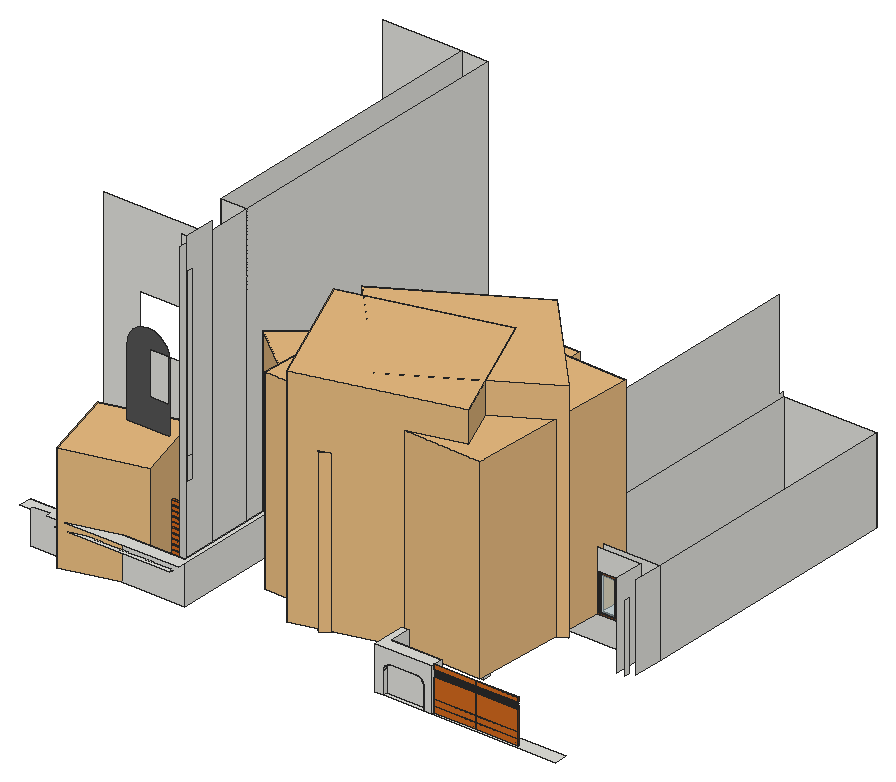
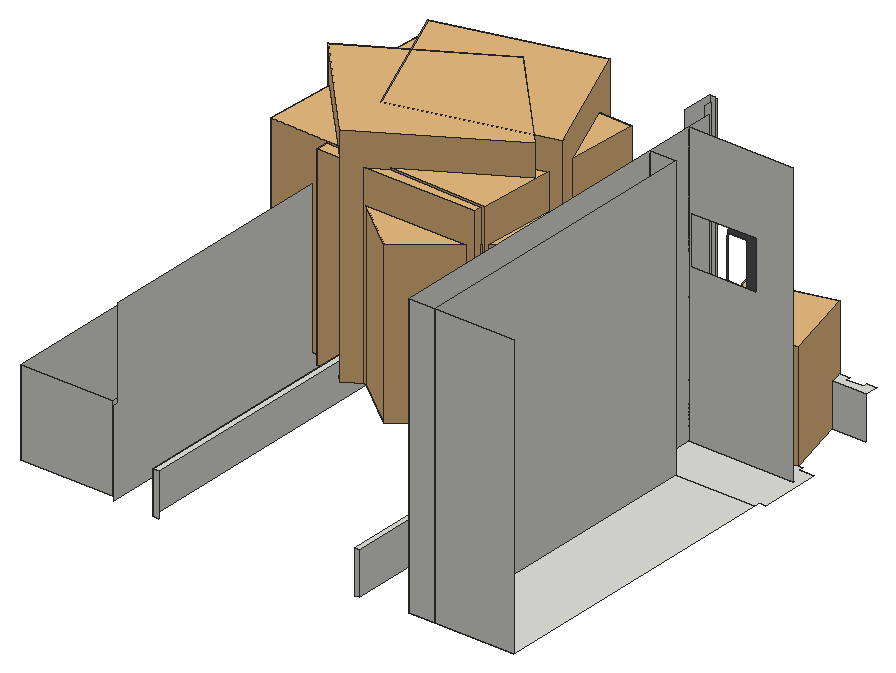
# SketchUp Ruby script. Lengths in inches.
U = 1.inch
M = Sketchup.active_model
def pt(a) = Geom::Point3d.new(a.map { |v| v * U })
def face(e, loops, mat)
  f = e.add_face(loops[0].map { |a| pt(a) })
  loops[1..].each { |l| e.add_face(l.map { |a| pt(a) }).erase! }
  f.material = f.back_material = mat if mat
  f
end
# faces: each face lists its corners as indices into pts; further lists are holes
def faces(e, pts, list, mat = nil) = list.each { |f| face(e, (f[0].is_a?(Array) ? f : [f]).map { |l| l.map { |i| pts[i] } }, mat) }
# xy, xz, yz: faces in a plane at the given z, y or x. An outline is a flat list of corners, or four numbers for a rectangle; further outlines are holes
def ring(l) = l.size == 4 ? [[l[0], l[1]], [l[2], l[1]], [l[2], l[3]], [l[0], l[3]]] : l.each_slice(2).to_a
def flat(e, list, mat, &to3) = list.each { |f| face(e, (f[0].is_a?(Array) ? f : [f]).map { |l| ring(l).map { |u, v| to3.(u, v) } }, mat) }
def xy(e, z, list, mat = nil) = flat(e, list, mat) { |x, y| [x, y, z] }
def xz(e, y, list, mat = nil) = flat(e, list, mat) { |x, z| [x, y, z] }
def yz(e, x, list, mat = nil) = flat(e, list, mat) { |y, z| [x, y, z] }
def lines(e, pts, list) = list.each { |a, b| e.add_line(pt(pts[a]), pt(pts[b])) }
# prism: a flat outline (further loops are holes) pulled along v
def prism(e, loops, v, mat = nil)
  f = face(e, loops, mat); d = Geom::Vector3d.new(v.map { |x| x * U })
  f.pushpull(f.normal.samedirection?(d) ? d.length : -d.length)
end
def box(e, o, s, mat = nil) = prism(e, [[o, [o[0] + s[0], o[1], o[2]], [o[0] + s[0], o[1] + s[1], o[2]], [o[0], o[1] + s[1], o[2]]]], [0, 0, s[2]], mat)
def at(x, y, z, deg = 0) = Geom::Transformation.translation(pt([x, y, z])) * Geom::Transformation.rotation(ORIGIN, Z_AXIS, deg.degrees)
def axes(o, x, y, z) = Geom::Transformation.new([*x, 0, *y, 0, *z, 0, *pt(o).to_a, 1])
def part(name) = M.definitions.add(name)
# library, detail: a bought-in or finely detailed component or shape, given as its bounding box
def library(name, o, s) = part(name).tap { |d| box(d.entities, o, s) }
def detail(e, o, s) = box(e.add_group.entities, o, s)
def put(e, d, t, mat = nil) = e.add_instance(d, t).tap { |i| i.material = mat if mat }
def group(e, t, mat = nil) = e.add_group.tap { |g| g.transformation = t; g.material = mat if mat }.entities
root = M.entities
M.materials.add("[0041_Chocolate]").color = [210, 105, 30]
M.materials.add("[Color M06]").color = [84, 84, 84]
M.materials.add("[Translucent Glass Safety]").color = [204, 235, 244]
M.materials["[Translucent Glass Safety]"].alpha = 0.5
M.materials.add("[Wood Veneer 01]").color = [120, 70, 37]
M.materials.add("[Wood Veneer 01]2").color = [94, 55, 29]
c1 = library("Palm tree",[-4.09,-4.52,0],[193.52,193.51,258.93])
c2 = part("Palm+Tree")
put(c2.entities,c1,at(25.51,-21.81,0,15))
c3 = library("Group\#287",[-33.32,-34.9375,32.67],[162.87,159.66,128.34])
c4 = library("Group\#288",[-10.45,-6.67,0],[121.7,116.61,164.95])
c5 = library("Group\#286",[-10.45,-6.67,0],[121.7,116.61,164.95])
c6 = library("Group\#284",[-10.45,-6.67,0],[121.7,116.61,164.95])
c7 = library("Group\#283",[-33.32,-34.9375,32.67],[162.87,159.66,128.34])
c8 = library("Group\#285",[-33.32,-34.9375,81.35],[162.87,159.66,79.66])
c9 = library("Group\#282",[-33.32,-34.9375,77.91],[162.87,159.66,83.1])
c10 = part("Palem Elek")
put(c10.entities,c3,axes([92.2,20.3,-29.73],[0.70711,0.70711,0],[-0.70711,0.70711,0],[0,0,0.91208]))
put(c10.entities,c4,axes([60.27,20.78,0],[1,0,0],[0,1,0],[0,0,0.85762]))
put(c10.entities,c5,at(25.45,60.83,0,-53.5))
put(c10.entities,c6,at(84.4375,135.48,0,-161.4))
put(c10.entities,c7,axes([38.54,105.7,-36.19],[-0.04013,-0.99919,0],[0.99919,-0.04013,0],[0,0,1.11001]))
put(c10.entities,c8,axes([57.15,96.51,-54.45],[-0.02003,-0.49872,0.02965],[0.4996,-0.02007,0],[0.00123,0.03065,0.51628]))
put(c10.entities,c9,axes([74.94,50.39,-54.06],[0.40095,0.29715,0.03075],[-0.29654,0.38966,0.10114],[0.04012,-0.11026,0.54246]))
c11 = part("palem elek\#1")
put(c11.entities,c10,at(-81.14,-74.56,-0.83))
c12 = part("Coqueiro")
put(c12.entities,c11,axes([83.17,89.39,9.5625],[0,1.1016,0],[-1.377,0,0],[0,0,1.39284]))
c13 = part("Slatted screen panel")
xy(c13.entities,0,[[0,0,255.91,1.97]],"[Wood Veneer 01]2")
xy(c13.entities,16.54,[[0,1.18,255.91,1.97]],"[Wood Veneer 01]2")
xy(c13.entities,16.93,[[0,0,255.91,1.18]],"[Wood Veneer 01]2")
xy(c13.entities,17.78,[[0,0,255.91,1.18]],"[Wood Veneer 01]2")
xy(c13.entities,34.45,[[0,0,255.91,1.18]],"[Wood Veneer 01]2")
xy(c13.entities,35.07,[[0,0,255.91,1.18]],"[Wood Veneer 01]2")
xy(c13.entities,89.37,[[0,0,255.91,1.97]],"[Wood Veneer 01]2")
xy(c13.entities,92.91,[[0,0,255.91,1.97]],"[Wood Veneer 01]2")
xy(c13.entities,94.49,[[0,0,255.91,1.97]],"[Wood Veneer 01]2")
xy(c13.entities,97.64,[[0,0,255.91,1.97]],"[Wood Veneer 01]2")
xy(c13.entities,99.21,[[0,0,255.91,1.97]],"[Wood Veneer 01]2")
xy(c13.entities,102.36,[[0,0,255.91,1.97]],"[Wood Veneer 01]2")
xy(c13.entities,103.9375,[[0,0,255.91,1.97]],"[Wood Veneer 01]2")
xy(c13.entities,107.48,[[0,0,255.91,1.97]],"[Wood Veneer 01]2")
xy(c13.entities,119.29,[[0,0,255.91,1.97]],"[Wood Veneer 01]2")
xz(c13.entities,0,[[0,0,255.91,16.93],[0,17.78,255.91,34.45],[0,35.07,255.91,89.37],[0,92.91,255.91,94.49],[0,97.64,255.91,99.21],
  [0,102.36,255.91,103.9375],[0,107.48,255.91,119.29]],"[0041_Chocolate]")
xz(c13.entities,1.18,[[0,16.54,255.91,16.93],[0,16.93,255.91,17.78],[0,34.45,255.91,35.07]],"[Wood Veneer 01]2")
xz(c13.entities,1.97,[[0,0,255.91,1.57],[0,1.57,255.91,5.51],[0,5.51,255.91,7.09],[0,7.09,255.91,11.8125],[0,11.8125,255.91,16.54],
  [0,16.54,255.91,19.69],[0,19.69,255.91,89.37],[0,92.91,255.91,94.49],[0,97.64,255.91,99.21],[0,102.36,255.91,103.9375],
  [0,107.48,255.91,109.84],[0,109.84,255.91,119.29]],"[Wood Veneer 01]2")
yz(c13.entities,0,[[0,0,1.97,1.57],[0,1.57,1.97,5.51],[0,5.51,1.97,7.09],[0,7.09,1.97,11.8125],[0,11.8125,0,16.93,1.18,16.93,1.18,16.54,1.97,16.54,1.97,11.8125],
  [1.18,16.54,1.97,19.69],[0,17.78,0,34.45,1.18,34.45,1.18,35.07,0,35.07,0,89.37,1.97,89.37,1.97,19.69,1.18,19.69,1.18,17.78],[0,92.91,1.97,94.49],[0,97.64,1.97,99.21],[0,102.36,1.97,103.9375],
  [0,107.48,1.97,109.84],[0,109.84,1.97,119.29]],"[Wood Veneer 01]2")
yz(c13.entities,255.91,[[0,0,1.97,1.57],[0,1.57,1.97,5.51],[0,5.51,1.97,7.09],[0,7.09,1.97,11.8125],[0,11.8125,1.97,11.8125,1.97,16.54,1.18,16.54,1.18,16.93,0,16.93],
  [1.18,16.54,1.97,19.69],[0,17.78,1.18,17.78,1.18,19.69,1.97,19.69,1.97,89.37,0,89.37,0,35.07,1.18,35.07,1.18,34.45,0,34.45],[0,92.91,1.97,94.49],[0,97.64,1.97,99.21],[0,102.36,1.97,103.9375],
  [0,107.48,1.97,109.84],[0,109.84,1.97,119.29]],"[Wood Veneer 01]2")
p = [[255.91,1.97,103.9375],[255.91,1.97,107.48],[0,1.97,107.48],[0,1.97,103.9375],[0,1.97,92.91],[0,1.97,89.37],
  [255.91,1.97,99.21],[255.91,1.97,102.36],[255.91,1.97,89.37],[255.91,1.97,92.91],[0,1.97,97.64],[0,1.97,94.49],
  [0,1.97,102.36],[0,1.97,99.21],[255.91,1.97,94.49],[255.91,1.97,97.64],[240.94,0,5.51],[240.94,1.97,5.51]]
lines(c13.entities,p,[[0,1],[2,3],[4,5],[6,7],[8,9],[10,11],[12,13],[14,15],[16,17]])
c14 = part("Group\#3")
g1 = group(c14.entities,at(0,0,0))
xy(g1,0,[[0,0,6,48]],"[Wood Veneer 01]")
xy(g1,4,[[0,4,1.8125,44],[1.8125,4,6,44]])
xy(g1,80,[[0,4,1.8125,44],[1.8125,4,6,44]])
xy(g1,84,[[0,0,6,48]],"[Wood Veneer 01]")
xz(g1,0,[[0,0,6,84]],"[Wood Veneer 01]")
xz(g1,4,[[0,4,1.8125,80],[1.8125,4,6,80]])
xz(g1,44,[[0,4,1.8125,80],[1.8125,4,6,80]])
xz(g1,48,[[0,0,6,84]],"[Wood Veneer 01]")
yz(g1,0,[[[0,0,48,84],[4,4,44,80]]],"[Wood Veneer 01]")
yz(g1,1.8125,[[4,4,44,80]],"[Translucent Glass Safety]")
yz(g1,6,[[[0,0,48,84],[4,4,44,80]]],"[Wood Veneer 01]")
g2 = group(c14.entities,at(0,48,0))
xy(g2,0,[[0,0,6,48]],"[Wood Veneer 01]")
xy(g2,4,[[0,4,1.8125,44],[1.8125,4,6,44]])
xy(g2,80,[[0,4,1.8125,44],[1.8125,4,6,44]])
xy(g2,84,[[0,0,6,48]],"[Wood Veneer 01]")
xz(g2,0,[[0,0,6,84]],"[Wood Veneer 01]")
xz(g2,4,[[0,4,1.8125,80],[1.8125,4,6,80]])
xz(g2,44,[[0,4,1.8125,80],[1.8125,4,6,80]])
xz(g2,48,[[0,0,6,84]],"[Wood Veneer 01]")
yz(g2,0,[[[0,0,48,84],[4,4,44,80]]],"[Wood Veneer 01]")
yz(g2,1.8125,[[4,4,44,80]],"[Translucent Glass Safety]")
yz(g2,6,[[[0,0,48,84],[4,4,44,80]]],"[Wood Veneer 01]")
xy(root,6.125,[[1930.49,889.52,1987.36,895.77],[1998.3,889.52,2173.1,908.02],[1476.02,971.36,1571.54,971.36,1571.54,983.34,1570.66,983.34,1570.66,992.96,1476.02,992.96],[1571.54,971.36,1577.46,983.34],[1475.52,983.34,1476.02,993.35],
  [1570.66,983.34,1571.54,993.35],[1571.54,983.34,1578.33,993.35],[1982.33,985.23,1995.33,996.48],[1476.02,992.96,1570.66,993.35],[[1476.02,993.35,1571.54,993.35,1571.54,1097.28,1423.34,1097.28,1423.34,1088.75,1414.82,1088.75,1414.82,1003.71,1436.06,1003.71,1436.06,996.48,1476.02,996.48],[1423.34,1012.23,1424.53,1088.75]],
  [1476.02,993.35,1476.02,996.48,1436.06,996.48,1436.06,1003.71,1424.53,1003.71,1424.53,1027.17,1571.54,1027.17,1571.54,993.35],[1476.02,993.35,1476.02,996.48,1436.06,996.48,1436.06,1003.71,1476.02,1003.71,1476.02,996.48,1571.54,996.48,1571.54,993.35],[1475.52,993.35,1476.02,996.48],[1571.54,993.35,1578.33,996.48],[1571.54,996.48,1578.33,1027.17],
  [1424.53,1027.17,1571.54,1028.46],[1423.34,1097.28,1534.54,1521.81],[1534.54,1097.28,1571.54,1521.81],[1989.57,1139.4,2119.65,1521.81]])
xy(root,11.08,[[1476.02,971.36,1577.46,972.36]],"[0041_Chocolate]")
xy(root,13.1875,[[1476.02,971.36,1577.46,972.36]],"[0041_Chocolate]")
xy(root,18.14,[[1476.02,971.36,1577.46,972.36]],"[0041_Chocolate]")
xy(root,20.25,[[1476.02,971.36,1577.46,972.36]],"[0041_Chocolate]")
xy(root,25.2,[[1476.02,971.36,1577.46,972.36]],"[0041_Chocolate]")
xy(root,27.3125,[[1476.02,971.36,1577.46,972.36]],"[0041_Chocolate]")
xy(root,32.27,[[1476.02,971.36,1577.46,972.36]],"[0041_Chocolate]")
xy(root,34.375,[[1476.02,971.36,1577.46,972.36]],"[0041_Chocolate]")
xy(root,39.33,[[1476.02,971.36,1577.46,972.36]],"[0041_Chocolate]")
xy(root,40.13,[[2018.31,1130.875,2065.93,1139.4]])
xy(root,41.4375,[[1476.02,971.36,1577.46,972.36]],"[0041_Chocolate]")
xy(root,46.39,[[1476.02,971.36,1577.46,972.36]],"[0041_Chocolate]")
xy(root,48,[[1941.42,889.52,1975.87,895.77]])
xy(root,48.5,[[1476.02,971.36,1577.46,972.36]],"[0041_Chocolate]")
xy(root,53.45,[[1476.02,971.36,1577.46,972.36]],"[0041_Chocolate]")
xy(root,55.1875,[[1467.3125,889.52,1467.3125,894.77,1468.9375,894.77,1468.9375,895.77,1469.6875,895.77,1469.6875,894.77,1472.9375,894.77,1472.9375,895.77,1473.6875,895.77,1473.6875,894.77,1476.9375,894.77,1476.9375,895.77,1477.6875,895.77,1477.6875,894.77,1480.9375,894.77,1480.9375,895.77,1481.6875,895.77,1481.6875,894.77,1484.9375,894.77,1484.9375,895.77,1485.6875,895.77,1485.6875,894.77,1488.9375,894.77,1488.9375,895.77,1489.6875,895.77,1489.6875,894.77,1492.9375,894.77,1492.9375,895.77,1493.6875,895.77,1493.6875,894.77,1496.9375,894.77,1496.9375,895.77,1497.6875,895.77,1497.6875,894.77,1500.9375,894.77,1500.9375,895.77,1501.6875,895.77,1501.6875,894.77,1504.9375,894.77,1504.9375,895.77,1505.6875,895.77,1505.6875,894.77,1508.9375,894.77,1508.9375,895.77,1509.6875,895.77,1509.6875,894.77,1512.9375,894.77,1512.9375,895.77,1513.6875,895.77,1513.6875,894.77,1516.9375,894.77,1516.9375,895.77,1517.6875,895.77,1517.6875,894.77,1520.9375,894.77,1520.9375,895.77,1521.6875,895.77,1521.6875,894.77,1524.9375,894.77,1524.9375,895.77,1525.6875,895.77,1525.6875,894.77,1528.9375,894.77,1528.9375,895.77,1529.6875,895.77,1529.6875,894.77,1532.9375,894.77,1532.9375,895.77,1533.6875,895.77,1533.6875,894.77,1536.9375,894.77,1536.9375,895.77,1537.6875,895.77,1537.6875,894.77,1540.9375,894.77,1540.9375,895.77,1541.6875,895.77,1541.6875,894.77,1544.9375,894.77,1544.9375,895.77,1545.6875,895.77,1545.6875,894.77,1548.9375,894.77,1548.9375,895.77,1549.6875,895.77,1549.6875,894.77,1552.9375,894.77,1552.9375,895.77,1553.6875,895.77,1553.6875,894.77,1556.9375,894.77,1556.9375,895.77,1557.6875,895.77,1557.6875,894.77,1560.9375,894.77,1560.9375,895.77,1561.6875,895.77,1561.6875,894.77,1564.9375,894.77,1564.9375,895.77,1565.6875,895.77,1565.6875,894.77,1568.9375,894.77,1568.9375,895.77,1569.6875,895.77,1569.6875,894.77,1572.9375,894.77,1572.9375,895.77,1573.6875,895.77,1573.6875,894.77,1576.9375,894.77,1576.9375,895.77,1577.6875,895.77,1577.6875,894.77,1580.9375,894.77,1580.9375,895.77,1581.6875,895.77,1581.6875,894.77,1584.9375,894.77,1584.9375,895.77,1585.6875,895.77,1585.6875,894.77,1588.9375,894.77,1588.9375,895.77,1589.6875,895.77,1589.6875,894.77,1592.9375,894.77,1592.9375,895.77,1593.6875,895.77,1593.6875,894.77,1596.9375,894.77,1596.9375,895.77,1597.6875,895.77,1597.6875,894.77,1600.9375,894.77,1600.9375,895.77,1601.6875,895.77,1601.6875,894.77,1604.9375,894.77,1604.9375,895.77,1605.6875,895.77,1605.6875,894.77,1608.9375,894.77,1608.9375,895.77,1609.6875,895.77,1609.6875,894.77,1612.9375,894.77,1612.9375,895.77,1613.6875,895.77,1613.6875,894.77,1616.9375,894.77,1616.9375,895.77,1617.6875,895.77,1617.6875,894.77,1620.9375,894.77,1620.9375,895.77,1621.6875,895.77,1621.6875,894.77,1624.9375,894.77,1624.9375,895.77,1625.6875,895.77,1625.6875,894.77,1628.9375,894.77,1628.9375,889.52]])
xy(root,55.5625,[[1476.02,971.36,1577.46,972.36]],"[0041_Chocolate]")
xy(root,60.52,[[1476.02,971.36,1577.46,972.36]],"[0041_Chocolate]")
xy(root,62.625,[[1476.02,971.36,1577.46,972.36]],"[0041_Chocolate]")
xy(root,66.125,[[1418.47,889.52,1431.6,889.52,1431.6,895.77,1455.91,895.77,1455.91,889.52,1641.83,889.52,1641.83,1529.04,1635.31,1529.04,1635.31,908.02,1418.47,908.02],[1918.83,889.52,1998.3,889.52,1998.3,908.02,1927.01,908.02,1927.01,1529.04,1918.83,1529.04]])
xy(root,67.58,[[1476.02,971.36,1577.46,972.36]],"[0041_Chocolate]")
xy(root,69.6875,[[1476.02,971.36,1577.46,972.36]],"[0041_Chocolate]")
xy(root,74.64,[[1476.02,971.36,1512.22,972.36],[1530.17,971.36,1577.46,972.36]],"[0041_Chocolate]")
xy(root,76.75,[[1476.02,971.36,1507.13,972.36],[1535.26,971.36,1577.46,972.36]],"[0041_Chocolate]")
xy(root,81.7,[[1476.02,971.36,1500.29,972.36],[1542.1,971.36,1577.46,972.36]],"[0041_Chocolate]")
xy(root,83.8125,[[1476.02,971.36,1498.61,972.36],[1543.78,971.36,1577.46,972.36]],"[0041_Chocolate]")
xy(root,88.77,[[1476.02,971.36,1495.08,972.36],[1547.3125,971.36,1577.46,972.36]],"[0041_Chocolate]")
xz(root,889.52,[[1918.83,6.125,1930.49,6.125,1930.49,37.07,1930.58,38.5,1930.86,39.9,1931.32,41.25,1931.95,42.53,1932.74,43.72,1933.6875,44.8,1934.76,45.74,1935.95,46.54,1937.23,47.17,1938.59,47.63,1939.99,47.91,1941.42,48,1975.87,48,1977.37,47.9,1978.84,47.61,1980.26,47.125,1981.61,46.46,1982.86,45.625,1983.99,44.63,1984.99,43.5,1985.82,42.25,1986.49,40.9,1986.97,39.48,1987.26,38.01,1987.36,36.51,1987.36,6.125,1998.3,6.125,1998.3,66.125,1918.83,66.125]])
xz(root,895.77,[[1930.49,6.125,1987.36,6.125,1987.36,36.51,1987.26,38.01,1986.97,39.48,1986.49,40.9,1985.82,42.25,1984.99,43.5,1983.99,44.63,1982.86,45.625,1981.61,46.46,1980.26,47.125,1978.84,47.61,1977.37,47.9,1975.87,48,1941.42,48,1939.99,47.91,1938.59,47.63,1937.23,47.17,1935.95,46.54,1934.76,45.74,1933.6875,44.8,1932.74,43.72,1931.95,42.53,1931.32,41.25,1930.86,39.9,1930.58,38.5,1930.49,37.07]])
xz(root,908.02,[[1418.47,6.125,1635.31,66.125],[1927.01,6.125,1998.3,66.125]])
xz(root,971.36,[[1476.02,6.125,1577.46,11.08],[1476.02,13.1875,1577.46,18.14],[1476.02,20.25,1577.46,25.2],[1476.02,27.3125,1577.46,32.27],[1476.02,34.375,1577.46,39.33],
  [1476.02,41.4375,1577.46,46.39],[1476.02,48.5,1577.46,53.45],[1476.02,55.5625,1577.46,60.52],[1476.02,62.625,1577.46,67.58],[1476.02,69.6875,1577.46,69.6875,1577.46,74.64,1530.17,74.64,1528.91,74.12,1521.2,73.1,1513.49,74.12,1512.22,74.64,1476.02,74.64],
  [1476.02,76.75,1507.13,76.75,1506.3,77.09,1500.29,81.7,1476.02,81.7],[1535.26,76.75,1577.46,76.75,1577.46,81.7,1542.1,81.7,1536.09,77.09],[1476.02,83.8125,1498.61,83.8125,1495.4,88,1495.08,88.77,1476.02,88.77],[1543.78,83.8125,1577.46,83.8125,1577.46,88.77,1547.3125,88.77,1546.99,88]],"[0041_Chocolate]")
xz(root,972.36,[[1476.02,11.08,1577.46,13.1875],[1476.02,18.14,1577.46,20.25],[1476.02,25.2,1577.46,27.3125],[1476.02,32.27,1577.46,34.375],[1476.02,39.33,1577.46,41.4375],
  [1476.02,46.39,1577.46,48.5],[1476.02,53.45,1577.46,55.5625],[1476.02,60.52,1577.46,62.625],[1476.02,67.58,1577.46,69.6875],[1476.02,74.64,1512.22,74.64,1507.13,76.75,1476.02,76.75],
  [1530.17,74.64,1577.46,74.64,1577.46,76.75,1535.26,76.75],[1476.02,81.7,1500.29,81.7,1500.13,81.83,1498.61,83.8125,1476.02,83.8125],[1542.1,81.7,1577.46,81.7,1577.46,83.8125,1543.78,83.8125,1542.26,81.83],[1476.02,88.77,1495.08,88.77,1494.21,90.875,1476.02,90.875],[1547.3125,88.77,1577.46,88.77,1577.46,90.875,1548.19,90.875]],"[0041_Chocolate]")
xz(root,983.34,[[1570.66,6.125,1571.54,126.125],[1571.54,6.125,1577.46,126.125],[1577.46,6.125,1578.33,6.125,1578.33,421.25,1571.54,421.25,1571.54,141.26,1577.46,141.26]])
xz(root,985.23,[[1982.33,6.125,1995.33,128.75]])
xz(root,986.55,[[[1521.2,73.1,1528.91,74.12,1530.17,74.64,1535.26,76.75,1536.09,77.09,1542.1,81.7,1542.26,81.83,1543.78,83.8125,1546.99,88,1547.3125,88.77,1548.19,90.875,1549.97,95.18,1550.05,95.83,1550.24,97.27,1525.8,97.27,1525.8,145.27,1550.98,145.27,1550.98,253.3125,1550.33,258.27,1550.05,260.375,1549.97,261.02,1548.19,265.33,1547.3125,267.4375,1546.99,268.21,1543.78,272.39,1542.26,274.375,1542.1,274.5,1536.09,279.11,1535.26,279.45,1530.17,281.5625,1528.91,282.09,1521.2,283.1,1513.49,282.09,1512.22,281.5625,1507.13,279.45,1506.3,279.11,1500.29,274.5,1500.13,274.375,1498.61,272.39,1495.4,268.21,1495.08,267.4375,1494.21,265.33,1492.42,261.02,1492.34,260.375,1492.06,258.27,1491.41,253.3125,1491.41,102.89,1492.06,97.9375,1492.34,95.83,1492.42,95.18,1494.21,90.875,1495.08,88.77,1495.4,88,1498.61,83.8125,1500.13,81.83,1500.29,81.7,1506.3,77.09,1507.13,76.75,1512.22,74.64,1513.49,74.12],[1523.64,196.89,1550.33,258.27]]],"[Color M06]")
xz(root,993.35,[[1476.02,6.125,1562.99,8.32],[1562.99,6.125,1570.66,8.32],[1570.66,6.125,1571.54,8.32],[1571.54,6.125,1578.33,8.32],[1476.02,8.32,1562.99,126.125],
  [1562.99,8.32,1570.66,109.9375],[1570.66,8.32,1571.54,109.9375]])
xz(root,996.48,[[1982.33,6.125,1995.33,128.75]])
xz(root,1028.46,[[[1424.53,6.125,1571.54,402.64],[1476.02,226.8,1568.84,295.72]]])
xz(root,1097.28,[[1534.54,6.125,1571.54,402.64]])
xz(root,1130.875,[[[1982.33,6.125,2100.82,126.125],[2018.31,40.13,2065.93,95.51]]])
xz(root,1139.4,[[1989.57,6.125,1998.09,126.125],[[1998.09,6.125,2119.65,126.125],[2018.31,40.13,2065.93,95.51]]])
xz(root,1521.81,[[1423.34,6.125,1534.54,402.64],[1534.54,6.125,1571.54,402.64],[1989.57,6.125,2119.65,126.125]])
xz(root,1529.04,[[1635.31,6.125,1641.83,66.125],[1918.83,6.125,1927.01,66.125]])
yz(root,1476.02,[[971.36,6.125,971.36,11.08,972.36,11.08,972.36,13.1875,971.36,13.1875,971.36,18.14,972.36,18.14,972.36,20.25,971.36,20.25,971.36,25.2,972.36,25.2,972.36,27.3125,971.36,27.3125,971.36,32.27,972.36,32.27,972.36,34.375,971.36,34.375,971.36,39.33,972.36,39.33,972.36,41.4375,971.36,41.4375,971.36,46.39,972.36,46.39,972.36,48.5,971.36,48.5,971.36,53.45,972.36,53.45,972.36,55.5625,971.36,55.5625,971.36,60.52,972.36,60.52,972.36,62.625,971.36,62.625,971.36,67.58,972.36,67.58,972.36,69.6875,971.36,69.6875,971.36,74.64,972.36,74.64,972.36,76.75,971.36,76.75,971.36,81.7,972.36,81.7,972.36,83.8125,971.36,83.8125,971.36,88.77,972.36,88.77,972.36,90.875,971.36,90.875,971.36,95.83,972.36,95.83,972.36,97.9375,971.36,97.9375,971.36,102.89,972.36,102.89,972.36,105,971.36,105,971.36,109.95,972.36,109.95,972.36,112.0625,971.36,112.0625,971.36,117.02,972.36,117.02,972.36,119.125,971.36,119.125,971.36,124.08,972.36,124.08,972.36,126.1875,971.36,126.1875,971.36,131.14,972.36,131.14,972.36,133.25,971.36,133.25,971.36,138.2,972.36,138.2,972.36,140.3125,971.36,140.3125,971.36,141.26,983.34,141.26,983.34,126.125,993.35,126.125,993.35,6.125]])
yz(root,1534.54,[[1097.28,6.125,1521.81,402.64]])
yz(root,1570.66,[[983.34,6.125,993.35,126.125]])
yz(root,1571.54,[[993.35,6.125,1028.46,402.64],[1028.46,6.125,1097.28,402.64],[1097.28,6.125,1521.81,402.64]])
yz(root,1577.46,[[971.36,6.125,983.34,6.125,983.34,141.26,993.35,141.26,993.35,411.82,972.36,411.82,972.36,405.64,971.36,405.64,971.36,400.6875,972.36,400.6875,972.36,398.77,971.36,398.77,971.36,393.8125,972.36,393.8125,972.36,391.89,971.36,391.89,971.36,386.9375,972.36,386.9375,972.36,385.02,971.36,385.02,971.36,380.0625,972.36,380.0625,972.36,378.14,971.36,378.14,971.36,373.1875,972.36,373.1875,972.36,371.27,971.36,371.27,971.36,366.3125,972.36,366.3125,972.36,364.2,971.36,364.2,971.36,359.25,972.36,359.25,972.36,357.14,971.36,357.14,971.36,352.1875,972.36,352.1875,972.36,350.08,971.36,350.08,971.36,345.125,972.36,345.125,972.36,343.02,971.36,343.02,971.36,338.0625,972.36,338.0625,972.36,335.95,971.36,335.95,971.36,331,972.36,331,972.36,328.89,971.36,328.89,971.36,323.9375,972.36,323.9375,972.36,321.83,971.36,321.83,971.36,316.875,972.36,316.875,972.36,314.77,971.36,314.77,971.36,309.8125,972.36,309.8125,972.36,307.7,971.36,307.7,971.36,302.75,972.36,302.75,972.36,300.64,971.36,300.64,971.36,295.6875,972.36,295.6875,972.36,293.58,971.36,293.58,971.36,288.625,972.36,288.625,972.36,286.52,971.36,286.52,971.36,281.5625,972.36,281.5625,972.36,279.45,971.36,279.45,971.36,274.5,972.36,274.5,972.36,272.39,971.36,272.39,971.36,267.4375,972.36,267.4375,972.36,265.33,971.36,265.33,971.36,260.375,972.36,260.375,972.36,258.27,971.36,258.27,971.36,253.3125,972.36,253.3125,972.36,251.2,971.36,251.2,971.36,246.25,972.36,246.25,972.36,244.14,971.36,244.14,971.36,239.1875,972.36,239.1875,972.36,237.08,971.36,237.08,971.36,232.125,972.36,232.125,972.36,230.02,971.36,230.02,971.36,225.0625,972.36,225.0625,972.36,222.95,971.36,222.95,971.36,218,972.36,218,972.36,215.89,971.36,215.89,971.36,210.9375,972.36,210.9375,972.36,208.83,971.36,208.83,971.36,203.875,972.36,203.875,972.36,201.77,971.36,201.77,971.36,196.8125,972.36,196.8125,972.36,194.7,971.36,194.7,971.36,189.75,972.36,189.75,972.36,187.64,971.36,187.64,971.36,182.6875,972.36,182.6875,972.36,180.58,971.36,180.58,971.36,175.625,972.36,175.625,972.36,173.52,971.36,173.52,971.36,168.5625,972.36,168.5625,972.36,166.45,971.36,166.45,971.36,161.5,972.36,161.5,972.36,159.39,971.36,159.39,971.36,154.4375,972.36,154.4375,972.36,152.33,971.36,152.33,971.36,147.375,972.36,147.375,972.36,145.27,971.36,145.27,971.36,140.3125,972.36,140.3125,972.36,138.2,971.36,138.2,971.36,133.25,972.36,133.25,972.36,131.14,971.36,131.14,971.36,126.1875,972.36,126.1875,972.36,124.08,971.36,124.08,971.36,119.125,972.36,119.125,972.36,117.02,971.36,117.02,971.36,112.0625,972.36,112.0625,972.36,109.95,971.36,109.95,971.36,105,972.36,105,972.36,102.89,971.36,102.89,971.36,97.9375,972.36,97.9375,972.36,95.83,971.36,95.83,971.36,90.875,972.36,90.875,972.36,88.77,971.36,88.77,971.36,83.8125,972.36,83.8125,972.36,81.7,971.36,81.7,971.36,76.75,972.36,76.75,972.36,74.64,971.36,74.64,971.36,69.6875,972.36,69.6875,972.36,67.58,971.36,67.58,971.36,62.625,972.36,62.625,972.36,60.52,971.36,60.52,971.36,55.5625,972.36,55.5625,972.36,53.45,971.36,53.45,971.36,48.5,972.36,48.5,972.36,46.39,971.36,46.39,971.36,41.4375,972.36,41.4375,972.36,39.33,971.36,39.33,971.36,34.375,972.36,34.375,972.36,32.27,971.36,32.27,971.36,27.3125,972.36,27.3125,972.36,25.2,971.36,25.2,971.36,20.25,972.36,20.25,972.36,18.14,971.36,18.14,971.36,13.1875,972.36,13.1875,972.36,11.08,971.36,11.08]])
yz(root,1578.33,[[983.34,6.125,1027.17,6.125,1027.17,421.25,983.34,421.25,983.34,376.875,993.35,376.875,993.35,109.9375,990,109.9375,985.91,110.21,983.34,110.72]])
yz(root,1635.31,[[908.02,6.125,1529.04,66.125]])
yz(root,1927.01,[[908.02,6.125,1529.04,66.125]])
yz(root,1930.49,[[889.52,6.125,895.77,37.07]])
yz(root,1982.33,[[985.23,6.125,985.23,128.75,989.28,128.75,989.28,126.125,996.48,126.125,996.48,6.125],[1130.875,6.125,1130.875,252.47,1521.81,252.47,1521.81,126.125,1529.04,126.125,1529.04,6.125]])
yz(root,1987.36,[[889.52,6.125,895.77,36.51]])
yz(root,1989.57,[[1139.4,6.125,1521.81,126.125]])
yz(root,1995.33,[[985.23,6.125,996.48,128.75]])
yz(root,1998.3,[[889.52,6.125,908.02,66.125]])
yz(root,2018.31,[[1130.875,40.13,1139.4,95.51]])
yz(root,2065.93,[[1130.875,40.13,1139.4,95.51]])
yz(root,2100.82,[[1088.75,6.125,1130.875,126.125]])
yz(root,2110.86,[[1088.75,6.125,1095.9375,101.1875]])
yz(root,2119.65,[[1097.28,6.125,1139.4,126.125],[1139.4,6.125,1521.81,126.125]])
p = [[1987.26,895.77,38.01],[1987.36,895.77,36.51],[1987.36,889.52,36.51],[1987.26,889.52,38.01],[1930.49,895.77,37.07],[1930.58,895.77,38.5],
  [1930.58,889.52,38.5],[1930.49,889.52,37.07],[1986.97,895.77,39.48],[1986.97,889.52,39.48],[1930.86,895.77,39.9],[1930.86,889.52,39.9],
  [1986.49,895.77,40.9],[1986.49,889.52,40.9],[1931.32,895.77,41.25],[1931.32,889.52,41.25],[1985.82,895.77,42.25],[1985.82,889.52,42.25],
  [1931.95,895.77,42.53],[1931.95,889.52,42.53],[1984.99,895.77,43.5],[1984.99,889.52,43.5],[1932.74,895.77,43.72],[1932.74,889.52,43.72],
  [1983.99,895.77,44.63],[1983.99,889.52,44.63],[1933.6875,895.77,44.8],[1933.6875,889.52,44.8],[1982.86,895.77,45.625],[1982.86,889.52,45.625],
  [1934.76,895.77,45.74],[1934.76,889.52,45.74],[1981.61,895.77,46.46],[1981.61,889.52,46.46],[1935.95,895.77,46.54],[1935.95,889.52,46.54],
  [1937.23,895.77,47.17],[1937.23,889.52,47.17],[1980.26,895.77,47.125],[1980.26,889.52,47.125],[1978.84,895.77,47.61],[1978.84,889.52,47.61],
  [1938.59,895.77,47.63],[1938.59,889.52,47.63],[1939.99,895.77,47.91],[1939.99,889.52,47.91],[1977.37,895.77,47.9],[1977.37,889.52,47.9],
  [1941.42,895.77,48],[1941.42,889.52,48],[1975.87,895.77,48],[1975.87,889.52,48],[1513.49,986.55,74.12],[1513.49,971.36,74.12],
  [1521.2,971.36,73.1],[1521.2,986.55,73.1],[1528.91,971.36,74.12],[1528.91,986.55,74.12],[1512.22,986.55,74.64],[1512.22,972.36,74.64],
  [1512.22,971.36,74.64],[1530.17,971.36,74.64],[1530.17,972.36,74.64],[1530.17,986.55,74.64],[1507.13,972.36,76.75],[1507.13,986.55,76.75],
  [1535.26,972.36,76.75],[1535.26,986.55,76.75],[1506.3,986.55,77.09],[1506.3,971.36,77.09],[1507.13,971.36,76.75],[1535.26,971.36,76.75],
  [1536.09,971.36,77.09],[1536.09,986.55,77.09],[1500.29,986.55,81.7],[1500.29,972.36,81.7],[1500.29,971.36,81.7],[1542.1,971.36,81.7],
  [1542.1,972.36,81.7],[1542.1,986.55,81.7],[1500.13,972.36,81.83],[1500.13,986.55,81.83],[1542.26,972.36,81.83],[1542.26,986.55,81.83],
  [1498.61,972.36,83.8125],[1498.61,986.55,83.8125],[1543.78,972.36,83.8125],[1543.78,986.55,83.8125],[1495.4,986.55,88],[1495.4,971.36,88],
  [1498.61,971.36,83.8125],[1543.78,971.36,83.8125],[1546.99,971.36,88],[1546.99,986.55,88],[1495.08,986.55,88.77],[1495.08,972.36,88.77],
  [1495.08,971.36,88.77],[1547.3125,971.36,88.77],[1547.3125,972.36,88.77],[1547.3125,986.55,88.77],[1494.21,972.36,90.875],[1494.21,986.55,90.875],
  [1548.19,972.36,90.875],[1548.19,986.55,90.875],[1476.02,1003.71,24.125],[1476.02,1003.71,6.125],[1476.02,1012.23,24.125]]
faces(root,p,[[0,1,2,3],[4,5,6,7],[8,0,3,9],[5,10,11,6],[12,8,9,13],[10,14,15,11],[16,12,13,17],[14,18,19,15],
  [20,16,17,21],[18,22,23,19],[24,20,21,25],[22,26,27,23],[28,24,25,29],[26,30,31,27],[32,28,29,33],[30,34,35,31],
  [34,36,37,35],[38,32,33,39],[40,38,39,41],[36,42,43,37],[42,44,45,43],[46,40,41,47],[44,48,49,45],[50,46,47,51]])
faces(root,p,[[52,53,54,55],[55,54,56,57],[58,59,60,53,52],[57,56,61,62,63],[64,59,58,65],[62,66,67,63],[68,69,70,64,65],[67,66,71,72,73],
  [74,75,76,69,68],[73,72,77,78,79],[80,75,74,81],[78,82,83,79],[84,80,81,85],[82,86,87,83],[88,89,90,84,85],[87,86,91,92,93],
  [94,95,96,89,88],[93,92,97,98,99],[100,95,94,101],[98,102,103,99]],"[Color M06]")
lines(root,p,[[104,105],[104,106]])
put(root,c2,axes([1457.92,903.83,6.125],[0.58344,0,0],[0,0.58344,0],[0,0,0.58344]),"[Color M06]")
put(root,c12,axes([1729.26,937.64,29.13],[1.38444,0,0],[0,1.38444,0],[0,0,1.38444]))
put(root,c13,axes([1998.4,892.77,6.125],[0.23355,0,0],[0,0.5124,0],[0,0,0.5124]),"[0041_Chocolate]")
put(root,c14,axes([2018.31,1133.76,40.13],[0,-0.48,0],[0.49609,0,0],[0,0,0.65923]))
put(root,c13,axes([2058.16,892.77,6.125],[0.23355,0,0],[0,0.5124,0],[0,0,0.5124]),"[0041_Chocolate]")
